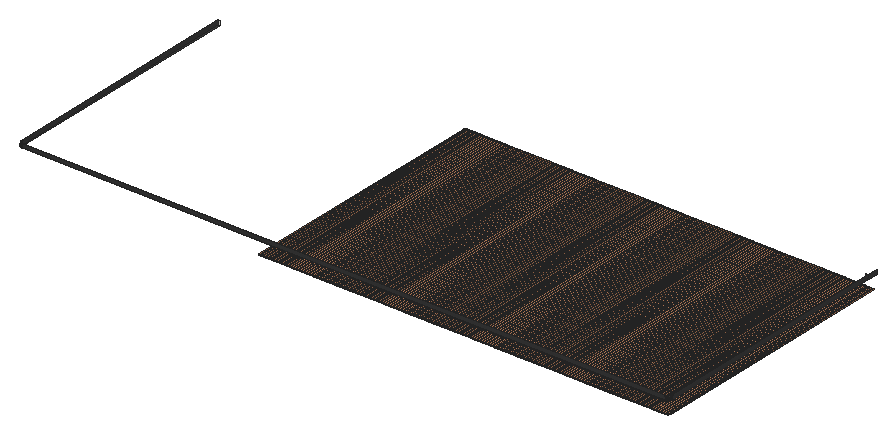
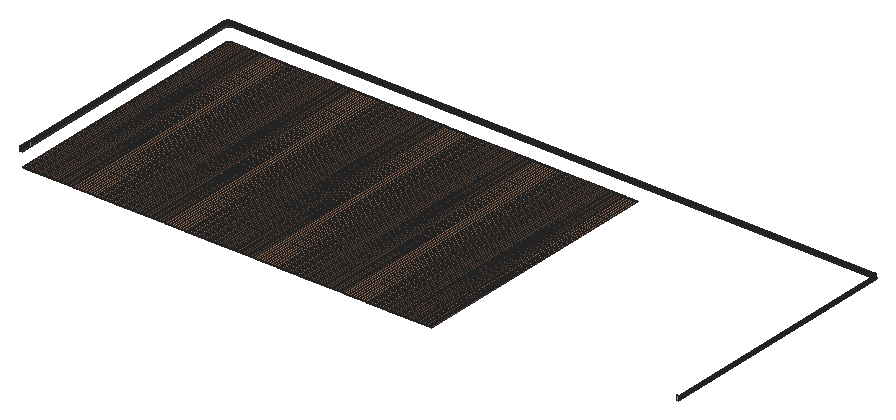
# SketchUp Ruby script. Lengths in inches.
U = 1.inch
M = Sketchup.active_model
def pt(a) = Geom::Point3d.new(a.map { |v| v * U })
def face(e, loops, mat)
  f = e.add_face(loops[0].map { |a| pt(a) })
  loops[1..].each { |l| e.add_face(l.map { |a| pt(a) }).erase! }
  f.material = f.back_material = mat if mat
  f
end
# faces: each face lists its corners as indices into pts; further lists are holes
def faces(e, pts, list, mat = nil) = list.each { |f| face(e, (f[0].is_a?(Array) ? f : [f]).map { |l| l.map { |i| pts[i] } }, mat) }
# xy, xz, yz: faces in a plane at the given z, y or x. An outline is a flat list of corners, or four numbers for a rectangle; further outlines are holes
def ring(l) = l.size == 4 ? [[l[0], l[1]], [l[2], l[1]], [l[2], l[3]], [l[0], l[3]]] : l.each_slice(2).to_a
def flat(e, list, mat, &to3) = list.each { |f| face(e, (f[0].is_a?(Array) ? f : [f]).map { |l| ring(l).map { |u, v| to3.(u, v) } }, mat) }
def xy(e, z, list, mat = nil) = flat(e, list, mat) { |x, y| [x, y, z] }
def xz(e, y, list, mat = nil) = flat(e, list, mat) { |x, z| [x, y, z] }
def yz(e, x, list, mat = nil) = flat(e, list, mat) { |y, z| [x, y, z] }
def lines(e, pts, list) = list.each { |a, b| e.add_line(pt(pts[a]), pt(pts[b])) }
# prism: a flat outline (further loops are holes) pulled along v
def prism(e, loops, v, mat = nil)
  f = face(e, loops, mat); d = Geom::Vector3d.new(v.map { |x| x * U })
  f.pushpull(f.normal.samedirection?(d) ? d.length : -d.length)
end
def box(e, o, s, mat = nil) = prism(e, [[o, [o[0] + s[0], o[1], o[2]], [o[0] + s[0], o[1] + s[1], o[2]], [o[0], o[1] + s[1], o[2]]]], [0, 0, s[2]], mat)
def at(x, y, z, deg = 0) = Geom::Transformation.translation(pt([x, y, z])) * Geom::Transformation.rotation(ORIGIN, Z_AXIS, deg.degrees)
def axes(o, x, y, z) = Geom::Transformation.new([*x, 0, *y, 0, *z, 0, *pt(o).to_a, 1])
def part(name) = M.definitions.add(name)
# library, detail: a bought-in or finely detailed component or shape, given as its bounding box
def library(name, o, s) = part(name).tap { |d| box(d.entities, o, s) }
def detail(e, o, s) = box(e.add_group.entities, o, s)
def put(e, d, t, mat = nil) = e.add_instance(d, t).tap { |i| i.material = mat if mat }
def group(e, t, mat = nil) = e.add_group.tap { |g| g.transformation = t; g.material = mat if mat }.entities
root = M.entities
M.materials.add("[Color M07]").color = [58, 58, 58]
M.materials.add("[Wood Veneer 02]").color = [190, 128, 91]
c1 = part("Group704\#1")
box(c1.entities,[-43,-63.59,0],[1,127.18,0.24])
c2 = part("Group705\#1")
box(c2.entities,[-41.7,-63.59,0],[1,127.18,0.24])
c3 = part("Group706\#1")
box(c3.entities,[-40.4,-63.59,0],[1,127.18,0.24])
c4 = part("Group707\#1")
box(c4.entities,[-39.1,-63.59,0],[1,127.18,0.24])
c5 = part("Group708\#1")
box(c5.entities,[-37.8,-63.59,0],[1,127.18,0.24])
c6 = part("Group709\#1")
box(c6.entities,[-36.5,-63.59,0],[1,127.18,0.24])
c7 = part("Group710\#1")
box(c7.entities,[-35.2,-63.59,0],[1,127.18,0.24])
c8 = part("Group711\#1")
box(c8.entities,[-33.9,-63.59,0],[1,127.18,0.24])
c9 = part("Group712\#1")
box(c9.entities,[-32.6,-63.59,0],[1,127.18,0.24])
c10 = part("Group713\#1")
box(c10.entities,[-31.3,-63.59,0],[1,127.18,0.24])
c11 = part("Group714\#1")
box(c11.entities,[-30,-63.59,0],[1,127.18,0.24])
c12 = part("Group715\#1")
box(c12.entities,[-28.7,-63.59,0],[1,127.18,0.24])
c13 = part("Group716\#1")
box(c13.entities,[-27.4,-63.59,0],[1,127.18,0.24])
c14 = part("Group717\#1")
box(c14.entities,[-26.1,-63.59,0],[1,127.18,0.24])
c15 = part("Group718\#1")
box(c15.entities,[-24.8,-63.59,0],[1,127.18,0.24])
c16 = part("Group719\#1")
box(c16.entities,[-23.5,-63.59,0],[1,127.18,0.24])
c17 = part("Group720\#1")
box(c17.entities,[-22.2,-63.59,0],[1,127.18,0.24])
c18 = part("Group721\#1")
box(c18.entities,[-20.9,-63.59,0],[1,127.18,0.24])
c19 = part("Group722\#1")
box(c19.entities,[-19.6,-63.59,0],[1,127.18,0.24])
c20 = part("Group723\#1")
box(c20.entities,[-18.3,-63.59,0],[1,127.18,0.24])
c21 = part("Group724\#1")
box(c21.entities,[-17,-63.59,0],[1,127.18,0.24])
c22 = part("Group725\#1")
box(c22.entities,[-15.7,-63.59,0],[1,127.18,0.24])
c23 = part("Group726\#1")
box(c23.entities,[-14.4,-63.59,0],[1,127.18,0.24])
c24 = part("Group727\#1")
box(c24.entities,[-13.1,-63.59,0],[1,127.18,0.24])
c25 = part("Group728\#1")
box(c25.entities,[-11.8,-63.59,0],[1,127.18,0.24])
c26 = part("Group729\#1")
box(c26.entities,[-10.5,-63.59,0],[1,127.18,0.24])
c27 = part("Group730\#1")
box(c27.entities,[-9.2,-63.59,0],[1,127.18,0.24])
c28 = part("Group731\#1")
box(c28.entities,[-7.9,-63.59,0],[1,127.18,0.24])
c29 = part("Group732\#1")
box(c29.entities,[-6.6,-63.59,0],[1,127.18,0.24])
c30 = part("Group733\#1")
box(c30.entities,[-5.3,-63.59,0],[1,127.18,0.24])
c31 = part("Group734\#1")
box(c31.entities,[-4,-63.59,0],[1,127.18,0.24])
c32 = part("Group735\#1")
box(c32.entities,[-2.7,-63.59,0],[1,127.18,0.24])
c33 = part("Group736\#1")
box(c33.entities,[-1.4,-63.59,0],[1,127.18,0.24])
c34 = part("Group737\#1")
box(c34.entities,[-0.1,-63.59,0],[1,127.18,0.24])
c35 = part("Group738\#1")
box(c35.entities,[1.2,-63.59,0],[1,127.18,0.24])
c36 = part("Group739\#1")
box(c36.entities,[2.5,-63.59,0],[1,127.18,0.24])
c37 = part("Group740\#1")
box(c37.entities,[3.8,-63.59,0],[1,127.18,0.24])
c38 = part("Group741\#1")
box(c38.entities,[5.1,-63.59,0],[1,127.18,0.24])
c39 = part("Group742\#1")
box(c39.entities,[6.4,-63.59,0],[1,127.18,0.24])
c40 = part("Group743\#1")
box(c40.entities,[7.7,-63.59,0],[1,127.18,0.24])
c41 = part("Group744\#1")
box(c41.entities,[9,-63.59,0],[1,127.18,0.24])
c42 = part("Group745\#1")
box(c42.entities,[10.3,-63.59,0],[1,127.18,0.24])
c43 = part("Group746\#1")
box(c43.entities,[11.6,-63.59,0],[1,127.18,0.24])
c44 = part("Group747\#1")
box(c44.entities,[12.9,-63.59,0],[1,127.18,0.24])
c45 = part("Group748\#1")
box(c45.entities,[14.2,-63.59,0],[1,127.18,0.24])
c46 = part("Group749\#1")
box(c46.entities,[15.5,-63.59,0],[1,127.18,0.24])
c47 = part("Group750\#1")
box(c47.entities,[16.8,-63.59,0],[1,127.18,0.24])
c48 = part("Group751\#1")
box(c48.entities,[18.1,-63.59,0],[1,127.18,0.24])
c49 = part("Group752\#1")
box(c49.entities,[19.4,-63.59,0],[1,127.18,0.24])
c50 = part("Group753\#1")
box(c50.entities,[20.7,-63.59,0],[1,127.18,0.24])
c51 = part("Group754\#1")
box(c51.entities,[22,-63.59,0],[1,127.18,0.24])
c52 = part("Group755\#1")
box(c52.entities,[23.3,-63.59,0],[1,127.18,0.24])
c53 = part("Group756\#1")
box(c53.entities,[24.6,-63.59,0],[1,127.18,0.24])
c54 = part("Group757\#1")
box(c54.entities,[25.9,-63.59,0],[1,127.18,0.24])
c55 = part("Group758\#1")
box(c55.entities,[27.2,-63.59,0],[1,127.18,0.24])
c56 = part("Group759\#1")
box(c56.entities,[28.5,-63.59,0],[1,127.18,0.24])
c57 = part("Group760\#1")
box(c57.entities,[29.8,-63.59,0],[1,127.18,0.24])
c58 = part("Group761\#1")
box(c58.entities,[31.1,-63.59,0],[1,127.18,0.24])
c59 = part("Group762\#1")
box(c59.entities,[32.4,-63.59,0],[1,127.18,0.24])
c60 = part("Group763\#1")
box(c60.entities,[33.7,-63.59,0],[1,127.18,0.24])
c61 = part("Group764\#1")
box(c61.entities,[35,-63.59,0],[1,127.18,0.24])
c62 = part("Group765\#1")
box(c62.entities,[36.3,-63.59,0],[1,127.18,0.24])
c63 = part("Group766\#1")
box(c63.entities,[37.6,-63.59,0],[1,127.18,0.24])
c64 = part("Group767\#1")
box(c64.entities,[38.9,-63.59,0],[1,127.18,0.24])
c65 = part("Group768\#1")
box(c65.entities,[40.2,-63.59,0],[1,127.18,0.24])
c66 = part("Group769\#1")
box(c66.entities,[41.5,-63.59,0],[1,127.18,0.24])
c67 = part("Group770\#1")
box(c67.entities,[42.8,-63.59,0],[1,127.18,0.24])
c68 = part("Group771\#1")
box(c68.entities,[44.1,-63.59,0],[1,127.18,0.24])
c69 = part("Group772\#1")
box(c69.entities,[45.4,-63.59,0],[1,127.18,0.24])
c70 = part("Group773\#1")
box(c70.entities,[46.7,-63.59,0],[1,127.18,0.24])
c71 = part("Group774\#1")
box(c71.entities,[48,-63.59,0],[1,127.18,0.24])
c72 = part("Group775\#1")
box(c72.entities,[49.3,-63.59,0],[1,127.18,0.24])
c73 = part("Group776\#1")
box(c73.entities,[50.6,-63.59,0],[1,127.18,0.24])
c74 = part("Group777\#1")
box(c74.entities,[51.9,-63.59,0],[1,127.18,0.24])
c75 = part("Group778\#1")
box(c75.entities,[53.2,-63.59,0],[1,127.18,0.24])
c76 = part("Group779\#1")
box(c76.entities,[54.5,-63.59,0],[1,127.18,0.24])
c77 = part("Group780\#1")
box(c77.entities,[55.8,-63.59,0],[1,127.18,0.24])
c78 = part("Group781\#1")
box(c78.entities,[57.1,-63.59,0],[1,127.18,0.24])
c79 = part("Group782\#1")
box(c79.entities,[58.4,-63.59,0],[1,127.18,0.24])
c80 = part("Group783\#1")
box(c80.entities,[59.7,-63.59,0],[1,127.18,0.24])
c81 = part("Group784\#1")
box(c81.entities,[61,-63.59,0],[1,127.18,0.24])
c82 = part("Group785\#1")
box(c82.entities,[62.3,-63.59,0],[1,127.18,0.24])
c83 = part("Group786\#1")
box(c83.entities,[63.6,-63.59,0],[1,127.18,0.24])
c84 = part("Group787\#1")
box(c84.entities,[64.9,-63.59,0],[1,127.18,0.24])
c85 = part("Group788\#1")
box(c85.entities,[66.2,-63.59,0],[1,127.18,0.24])
c86 = part("Group789\#1")
box(c86.entities,[67.5,-63.59,0],[1,127.18,0.24])
c87 = part("Group790\#1")
box(c87.entities,[68.8,-63.59,0],[1,127.18,0.24])
c88 = part("Group791\#1")
box(c88.entities,[70.1,-63.59,0],[1,127.18,0.24])
c89 = part("Group792\#1")
box(c89.entities,[71.4,-63.59,0],[1,127.18,0.24])
c90 = part("Group793\#1")
box(c90.entities,[72.7,-63.59,0],[1,127.18,0.24])
c91 = part("Group794\#1")
box(c91.entities,[74,-63.59,0],[1,127.18,0.24])
c92 = part("Group795\#1")
box(c92.entities,[75.3,-63.59,0],[1,127.18,0.24])
c93 = part("Group796\#1")
box(c93.entities,[76.6,-63.59,0],[1,127.18,0.24])
c94 = part("Group797\#1")
box(c94.entities,[77.9,-63.59,0],[1,127.18,0.24])
c95 = part("Group798\#1")
box(c95.entities,[79.2,-63.59,0],[1,127.18,0.24])
c96 = part("Group799\#1")
box(c96.entities,[80.5,-63.59,0],[1,127.18,0.24])
c97 = part("Group800\#1")
box(c97.entities,[81.8,-63.59,0],[1,127.18,0.24])
c98 = part("Group801\#1")
box(c98.entities,[83.1,-63.59,0],[1,127.18,0.24])
c99 = part("Group802\#1")
box(c99.entities,[84.4,-63.59,0],[1,127.18,0.24])
c100 = part("Group803\#1")
box(c100.entities,[85.7,-63.59,0],[1,127.18,0.24])
c101 = part("Group804\#1")
box(c101.entities,[87,-63.59,0],[1,127.18,0.24])
c102 = part("Group805\#1")
box(c102.entities,[88.3,-63.59,0],[1,127.18,0.24])
c103 = part("Group806\#1")
box(c103.entities,[89.6,-63.59,0],[1,127.18,0.24])
c104 = part("Group807\#1")
box(c104.entities,[90.9,-63.59,0],[1,127.18,0.24])
c105 = part("Group808\#1")
box(c105.entities,[92.2,-63.59,0],[1,127.18,0.24])
c106 = part("Group809\#1")
box(c106.entities,[93.5,-63.59,0],[1,127.18,0.24])
c107 = part("Group810\#1")
box(c107.entities,[94.8,-63.59,0],[1,127.18,0.24])
c108 = part("Group811\#1")
box(c108.entities,[96.1,-63.59,0],[1,127.18,0.24])
c109 = part("Group812\#1")
box(c109.entities,[97.4,-63.59,0],[1,127.18,0.24])
c110 = part("Group813\#1")
box(c110.entities,[98.7,-63.59,0],[1,127.18,0.24])
c111 = part("Group814\#1")
box(c111.entities,[100,-63.59,0],[1,127.18,0.24])
c112 = part("Group815\#1")
box(c112.entities,[101.3,-63.59,0],[1,127.18,0.24])
c113 = part("Group816\#1")
box(c113.entities,[102.6,-63.59,0],[1,127.18,0.24])
c114 = part("Group817\#1")
box(c114.entities,[103.9,-63.59,0],[1,127.18,0.24])
c115 = part("Group818\#1")
box(c115.entities,[105.2,-63.59,0],[1,127.18,0.24])
c116 = part("Group819\#1")
box(c116.entities,[106.5,-63.59,0],[1,127.18,0.24])
c117 = part("Group820\#1")
box(c117.entities,[107.8,-63.59,0],[1,127.18,0.24])
c118 = part("Group821\#1")
box(c118.entities,[109.1,-63.59,0],[1,127.18,0.24])
c119 = part("Group822\#1")
box(c119.entities,[110.4,-63.59,0],[1,127.18,0.24])
c120 = part("Group823\#1")
box(c120.entities,[111.7,-63.59,0],[1,127.18,0.24])
c121 = part("Group824\#1")
box(c121.entities,[113,-63.59,0],[1,127.18,0.24])
c122 = part("Group825\#1")
box(c122.entities,[114.3,-63.59,0],[1,127.18,0.24])
c123 = part("Group826\#1")
box(c123.entities,[115.6,-63.59,0],[1,127.18,0.24])
c124 = part("Group827\#1")
box(c124.entities,[116.9,-63.59,0],[1,127.18,0.24])
c125 = part("Group828\#1")
box(c125.entities,[118.2,-63.59,0],[1,127.18,0.24])
c126 = part("Group829\#1")
box(c126.entities,[119.5,-63.59,0],[1,127.18,0.24])
c127 = part("Group830\#1")
box(c127.entities,[120.8,-63.59,0],[1,127.18,0.24])
c128 = part("Group831\#1")
box(c128.entities,[122.1,-63.59,0],[1,127.18,0.24])
c129 = part("Group832\#1")
box(c129.entities,[123.4,-63.59,0],[1,127.18,0.24])
c130 = part("Group833\#1")
box(c130.entities,[124.7,-63.59,0],[1,127.18,0.24])
c131 = part("Group834\#1")
box(c131.entities,[126,-63.59,0],[1,127.18,0.24])
c132 = part("Group835\#1")
box(c132.entities,[127.3,-63.59,0],[1,127.18,0.24])
c133 = part("Group836\#1")
box(c133.entities,[128.6,-63.59,0],[1,127.18,0.24])
c134 = part("Group837\#1")
box(c134.entities,[129.9,-63.59,0],[1,127.18,0.24])
c135 = part("Group838\#1")
box(c135.entities,[131.2,-63.59,0],[1,127.18,0.24])
c136 = part("Group839\#1")
box(c136.entities,[132.5,-63.59,0],[1,127.18,0.24])
c137 = part("Group840\#1")
box(c137.entities,[133.8,-63.59,0],[1,127.18,0.24])
c138 = part("Group841\#1")
box(c138.entities,[135.1,-63.59,0],[1,127.18,0.24])
c139 = part("Group842\#1")
box(c139.entities,[136.4,-63.59,0],[1,127.18,0.24])
c140 = part("Group843\#1")
box(c140.entities,[137.7,-63.59,0],[1,127.18,0.24])
c141 = part("Group844\#1")
box(c141.entities,[139,-63.59,0],[1,127.18,0.24])
c142 = part("Group845\#1")
box(c142.entities,[140.3,-63.59,0],[1,127.18,0.24])
c143 = part("Group846\#1")
box(c143.entities,[141.6,-63.59,0],[1,127.18,0.24])
c144 = part("Group847\#1")
box(c144.entities,[142.9,-63.59,0],[1,127.18,0.24])
c145 = part("Group848\#1")
box(c145.entities,[144.2,-63.59,0],[1,127.18,0.24])
c146 = part("Group849\#1")
box(c146.entities,[145.5,-63.59,0],[1,127.18,0.24])
c147 = part("Group850\#1")
box(c147.entities,[146.8,-63.59,0],[1,127.18,0.24])
c148 = part("Group851\#1")
box(c148.entities,[148.1,-63.59,0],[1,127.18,0.24])
c149 = part("Group852\#1")
box(c149.entities,[149.4,-63.59,0],[1,127.18,0.24])
c150 = part("Group853\#1")
box(c150.entities,[150.7,-63.59,0],[1,127.18,0.24])
c151 = part("Group854\#1")
box(c151.entities,[152,-63.59,0],[1,127.18,0.24])
c152 = part("Group855\#1")
box(c152.entities,[153.3,-63.59,0],[1,127.18,0.24])
c153 = part("Group856\#1")
box(c153.entities,[154.6,-63.59,0],[1,127.18,0.24])
c154 = part("Group857\#1")
box(c154.entities,[155.9,-63.59,0],[1,127.18,0.24])
c155 = part("Group858\#1")
xy(c155.entities,0,[[157.2,-63.59,157.2,63.59,158.2,63.59,158.2,-63.57,157.94,-63.59]])
xy(c155.entities,0.24,[[157.2,-63.59,157.94,-63.59,158.2,-63.57,158.2,63.59,157.2,63.59]])
xz(c155.entities,63.59,[[157.2,0,158.2,0.24]])
yz(c155.entities,157.2,[[-63.59,0,63.59,0.24]])
yz(c155.entities,158.2,[[-63.57,0,63.59,0.24]])
c156 = part("Group859\#1")
xy(c156.entities,0,[[158.5,-63.54,158.5,63.59,159.5,63.59,159.5,-63.06,159.49,-63.08,159.09,-63.37,158.57,-63.54]])
xy(c156.entities,0.24,[[158.5,-63.54,158.57,-63.54,159.09,-63.37,159.49,-63.08,159.5,-63.06,159.5,63.59,158.5,63.59]])
xz(c156.entities,63.59,[[158.5,0,159.5,0.24]])
yz(c156.entities,158.5,[[-63.54,0,63.59,0.24]])
yz(c156.entities,159.5,[[-63.06,0,63.59,0.24]])
c157 = part("Group860\#1")
xy(c157.entities,0,[[159.8,-62.59,159.8,63.59,160,63.59,160,-61.54,159.94,-62.16]])
xy(c157.entities,0.24,[[159.8,-62.59,159.94,-62.16,160,-61.54,160,63.59,159.8,63.59]])
yz(c157.entities,159.8,[[-62.59,0,63.59,0.24]])
xy(root,133,[[2.06,0,1.43,0.03,0.91,0.11,0.51,0.25,0.23,0.44,0.06,0.69,0,1,0,123.1875,1,123.1875,1,3.06,1.06,2.43,1.23,1.91,1.51,1.51,1.91,1.23,2.43,1.06,3.06,1,318.94,1,319.57,1.06,320.09,1.23,320.49,1.51,320.77,1.91,320.94,2.43,321,3.06,321,123.1875,322,123.1875,322,2.06,321.97,1.43,321.89,0.91,321.75,0.51,321.56,0.23,321.31,0.06,321,0],[321,123.1875,322,128.1875]],"[Color M07]")
xz(root,0,[[2.06,133,321,133,319.94,135,2.06,135]],"[Color M07]")
xz(root,123.1875,[[0,133,1,135],[321,133,322,135]])
yz(root,0,[[1,133,2.06,135,123.1875,135,123.1875,133]],"[Color M07]")
yz(root,322,[[2.06,133,123.1875,135],[123.1875,133,128.1875,135]],"[Color M07]")
p = [[0.91,0.11,133],[1.43,0.03,133],[0.91,0.23,135],[1.43,0.06,135],[2.06,0,133],[2.06,0,135],
  [321.31,0.06,133],[320.57,0.06,135],[319.94,0,135],[321,0,133],[0.51,0.51,135],[0.51,0.25,133],
  [321.56,0.23,133],[321.09,0.23,135],[321.75,0.51,133],[321.49,0.51,135],[0.23,0.91,135],[0.23,0.44,133],
  [0.06,1.43,135],[0.06,0.69,133],[321.89,0.91,133],[321.77,0.91,135],[0,2.06,135],[0,1,133],
  [321.97,1.43,133],[321.94,1.43,135],[322,2.06,133],[322,2.06,135]]
faces(root,p,[[0,1,2],[1,3,2],[4,5,3],[1,4,3],[6,7,8],[9,6,8],[0,2,10],[11,0,10],
  [12,13,7],[6,12,7],[14,15,13],[12,14,13],[11,10,16],[17,11,16],[17,16,18],[19,17,18],
  [20,21,15],[14,20,15],[19,18,22],[23,19,22],[20,24,21],[24,25,21],[26,27,25],[24,26,25]],"[Color M07]")
put(root,c1,at(161,64.59,126),"[Wood Veneer 02]")
put(root,c2,at(161,64.59,126),"[Wood Veneer 02]")
put(root,c3,at(161,64.59,126),"[Wood Veneer 02]")
put(root,c4,at(161,64.59,126),"[Wood Veneer 02]")
put(root,c5,at(161,64.59,126),"[Wood Veneer 02]")
put(root,c6,at(161,64.59,126),"[Wood Veneer 02]")
put(root,c7,at(161,64.59,126),"[Wood Veneer 02]")
put(root,c8,at(161,64.59,126),"[Wood Veneer 02]")
put(root,c9,at(161,64.59,126),"[Wood Veneer 02]")
put(root,c10,at(161,64.59,126),"[Wood Veneer 02]")
put(root,c11,at(161,64.59,126),"[Wood Veneer 02]")
put(root,c12,at(161,64.59,126),"[Wood Veneer 02]")
put(root,c13,at(161,64.59,126),"[Wood Veneer 02]")
put(root,c14,at(161,64.59,126),"[Wood Veneer 02]")
put(root,c15,at(161,64.59,126),"[Wood Veneer 02]")
put(root,c16,at(161,64.59,126),"[Wood Veneer 02]")
put(root,c17,at(161,64.59,126),"[Wood Veneer 02]")
put(root,c18,at(161,64.59,126),"[Wood Veneer 02]")
put(root,c19,at(161,64.59,126),"[Wood Veneer 02]")
put(root,c20,at(161,64.59,126),"[Wood Veneer 02]")
put(root,c21,at(161,64.59,126),"[Wood Veneer 02]")
put(root,c22,at(161,64.59,126),"[Wood Veneer 02]")
put(root,c23,at(161,64.59,126),"[Wood Veneer 02]")
put(root,c24,at(161,64.59,126),"[Wood Veneer 02]")
put(root,c25,at(161,64.59,126),"[Wood Veneer 02]")
put(root,c26,at(161,64.59,126),"[Wood Veneer 02]")
put(root,c27,at(161,64.59,126),"[Wood Veneer 02]")
put(root,c28,at(161,64.59,126),"[Wood Veneer 02]")
put(root,c29,at(161,64.59,126),"[Wood Veneer 02]")
put(root,c30,at(161,64.59,126),"[Wood Veneer 02]")
put(root,c31,at(161,64.59,126),"[Wood Veneer 02]")
put(root,c32,at(161,64.59,126),"[Wood Veneer 02]")
put(root,c33,at(161,64.59,126),"[Wood Veneer 02]")
put(root,c34,at(161,64.59,126),"[Wood Veneer 02]")
put(root,c35,at(161,64.59,126),"[Wood Veneer 02]")
put(root,c36,at(161,64.59,126),"[Wood Veneer 02]")
put(root,c37,at(161,64.59,126),"[Wood Veneer 02]")
put(root,c38,at(161,64.59,126),"[Wood Veneer 02]")
put(root,c39,at(161,64.59,126),"[Wood Veneer 02]")
put(root,c40,at(161,64.59,126),"[Wood Veneer 02]")
put(root,c41,at(161,64.59,126),"[Wood Veneer 02]")
put(root,c42,at(161,64.59,126),"[Wood Veneer 02]")
put(root,c43,at(161,64.59,126),"[Wood Veneer 02]")
put(root,c44,at(161,64.59,126),"[Wood Veneer 02]")
put(root,c45,at(161,64.59,126),"[Wood Veneer 02]")
put(root,c46,at(161,64.59,126),"[Wood Veneer 02]")
put(root,c47,at(161,64.59,126),"[Wood Veneer 02]")
put(root,c48,at(161,64.59,126),"[Wood Veneer 02]")
put(root,c49,at(161,64.59,126),"[Wood Veneer 02]")
put(root,c50,at(161,64.59,126),"[Wood Veneer 02]")
put(root,c51,at(161,64.59,126),"[Wood Veneer 02]")
put(root,c52,at(161,64.59,126),"[Wood Veneer 02]")
put(root,c53,at(161,64.59,126),"[Wood Veneer 02]")
put(root,c54,at(161,64.59,126),"[Wood Veneer 02]")
put(root,c55,at(161,64.59,126),"[Wood Veneer 02]")
put(root,c56,at(161,64.59,126),"[Wood Veneer 02]")
put(root,c57,at(161,64.59,126),"[Wood Veneer 02]")
put(root,c58,at(161,64.59,126),"[Wood Veneer 02]")
put(root,c59,at(161,64.59,126),"[Wood Veneer 02]")
put(root,c60,at(161,64.59,126),"[Wood Veneer 02]")
put(root,c61,at(161,64.59,126),"[Wood Veneer 02]")
put(root,c62,at(161,64.59,126),"[Wood Veneer 02]")
put(root,c63,at(161,64.59,126),"[Wood Veneer 02]")
put(root,c64,at(161,64.59,126),"[Wood Veneer 02]")
put(root,c65,at(161,64.59,126),"[Wood Veneer 02]")
put(root,c66,at(161,64.59,126),"[Wood Veneer 02]")
put(root,c67,at(161,64.59,126),"[Wood Veneer 02]")
put(root,c68,at(161,64.59,126),"[Wood Veneer 02]")
put(root,c69,at(161,64.59,126),"[Wood Veneer 02]")
put(root,c70,at(161,64.59,126),"[Wood Veneer 02]")
put(root,c71,at(161,64.59,126),"[Wood Veneer 02]")
put(root,c72,at(161,64.59,126),"[Wood Veneer 02]")
put(root,c73,at(161,64.59,126),"[Wood Veneer 02]")
put(root,c74,at(161,64.59,126),"[Wood Veneer 02]")
put(root,c75,at(161,64.59,126),"[Wood Veneer 02]")
put(root,c76,at(161,64.59,126),"[Wood Veneer 02]")
put(root,c77,at(161,64.59,126),"[Wood Veneer 02]")
put(root,c78,at(161,64.59,126),"[Wood Veneer 02]")
put(root,c79,at(161,64.59,126),"[Wood Veneer 02]")
put(root,c80,at(161,64.59,126),"[Wood Veneer 02]")
put(root,c81,at(161,64.59,126),"[Wood Veneer 02]")
put(root,c82,at(161,64.59,126),"[Wood Veneer 02]")
put(root,c83,at(161,64.59,126),"[Wood Veneer 02]")
put(root,c84,at(161,64.59,126),"[Wood Veneer 02]")
put(root,c85,at(161,64.59,126),"[Wood Veneer 02]")
put(root,c86,at(161,64.59,126),"[Wood Veneer 02]")
put(root,c87,at(161,64.59,126),"[Wood Veneer 02]")
put(root,c88,at(161,64.59,126),"[Wood Veneer 02]")
put(root,c89,at(161,64.59,126),"[Wood Veneer 02]")
put(root,c90,at(161,64.59,126),"[Wood Veneer 02]")
put(root,c91,at(161,64.59,126),"[Wood Veneer 02]")
put(root,c92,at(161,64.59,126),"[Wood Veneer 02]")
put(root,c93,at(161,64.59,126),"[Wood Veneer 02]")
put(root,c94,at(161,64.59,126),"[Wood Veneer 02]")
put(root,c95,at(161,64.59,126),"[Wood Veneer 02]")
put(root,c96,at(161,64.59,126),"[Wood Veneer 02]")
put(root,c97,at(161,64.59,126),"[Wood Veneer 02]")
put(root,c98,at(161,64.59,126),"[Wood Veneer 02]")
put(root,c99,at(161,64.59,126),"[Wood Veneer 02]")
put(root,c100,at(161,64.59,126),"[Wood Veneer 02]")
put(root,c101,at(161,64.59,126),"[Wood Veneer 02]")
put(root,c102,at(161,64.59,126),"[Wood Veneer 02]")
put(root,c103,at(161,64.59,126),"[Wood Veneer 02]")
put(root,c104,at(161,64.59,126),"[Wood Veneer 02]")
put(root,c105,at(161,64.59,126),"[Wood Veneer 02]")
put(root,c106,at(161,64.59,126),"[Wood Veneer 02]")
put(root,c107,at(161,64.59,126),"[Wood Veneer 02]")
put(root,c108,at(161,64.59,126),"[Wood Veneer 02]")
put(root,c109,at(161,64.59,126),"[Wood Veneer 02]")
put(root,c110,at(161,64.59,126),"[Wood Veneer 02]")
put(root,c111,at(161,64.59,126),"[Wood Veneer 02]")
put(root,c112,at(161,64.59,126),"[Wood Veneer 02]")
put(root,c113,at(161,64.59,126),"[Wood Veneer 02]")
put(root,c114,at(161,64.59,126),"[Wood Veneer 02]")
put(root,c115,at(161,64.59,126),"[Wood Veneer 02]")
put(root,c116,at(161,64.59,126),"[Wood Veneer 02]")
put(root,c117,at(161,64.59,126),"[Wood Veneer 02]")
put(root,c118,at(161,64.59,126),"[Wood Veneer 02]")
put(root,c119,at(161,64.59,126),"[Wood Veneer 02]")
put(root,c120,at(161,64.59,126),"[Wood Veneer 02]")
put(root,c121,at(161,64.59,126),"[Wood Veneer 02]")
put(root,c122,at(161,64.59,126),"[Wood Veneer 02]")
put(root,c123,at(161,64.59,126),"[Wood Veneer 02]")
put(root,c124,at(161,64.59,126),"[Wood Veneer 02]")
put(root,c125,at(161,64.59,126),"[Wood Veneer 02]")
put(root,c126,at(161,64.59,126),"[Wood Veneer 02]")
put(root,c127,at(161,64.59,126),"[Wood Veneer 02]")
put(root,c128,at(161,64.59,126),"[Wood Veneer 02]")
put(root,c129,at(161,64.59,126),"[Wood Veneer 02]")
put(root,c130,at(161,64.59,126),"[Wood Veneer 02]")
put(root,c131,at(161,64.59,126),"[Wood Veneer 02]")
put(root,c132,at(161,64.59,126),"[Wood Veneer 02]")
put(root,c133,at(161,64.59,126),"[Wood Veneer 02]")
put(root,c134,at(161,64.59,126),"[Wood Veneer 02]")
put(root,c135,at(161,64.59,126),"[Wood Veneer 02]")
put(root,c136,at(161,64.59,126),"[Wood Veneer 02]")
put(root,c137,at(161,64.59,126),"[Wood Veneer 02]")
put(root,c138,at(161,64.59,126),"[Wood Veneer 02]")
put(root,c139,at(161,64.59,126),"[Wood Veneer 02]")
put(root,c140,at(161,64.59,126),"[Wood Veneer 02]")
put(root,c141,at(161,64.59,126),"[Wood Veneer 02]")
put(root,c142,at(161,64.59,126),"[Wood Veneer 02]")
put(root,c143,at(161,64.59,126),"[Wood Veneer 02]")
put(root,c144,at(161,64.59,126),"[Wood Veneer 02]")
put(root,c145,at(161,64.59,126),"[Wood Veneer 02]")
put(root,c146,at(161,64.59,126),"[Wood Veneer 02]")
put(root,c147,at(161,64.59,126),"[Wood Veneer 02]")
put(root,c148,at(161,64.59,126),"[Wood Veneer 02]")
put(root,c149,at(161,64.59,126),"[Wood Veneer 02]")
put(root,c150,at(161,64.59,126),"[Wood Veneer 02]")
put(root,c151,at(161,64.59,126),"[Wood Veneer 02]")
put(root,c152,at(161,64.59,126),"[Wood Veneer 02]")
put(root,c153,at(161,64.59,126),"[Wood Veneer 02]")
put(root,c154,at(161,64.59,126),"[Wood Veneer 02]")
put(root,c155,at(161,64.59,126),"[Wood Veneer 02]")
put(root,c156,at(161,64.59,126),"[Wood Veneer 02]")
put(root,c157,at(161,64.59,126),"[Wood Veneer 02]")
